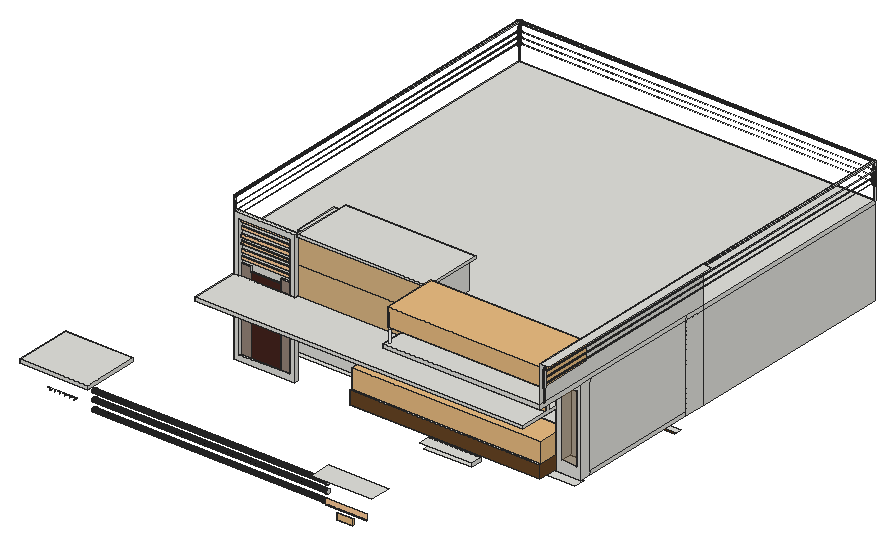
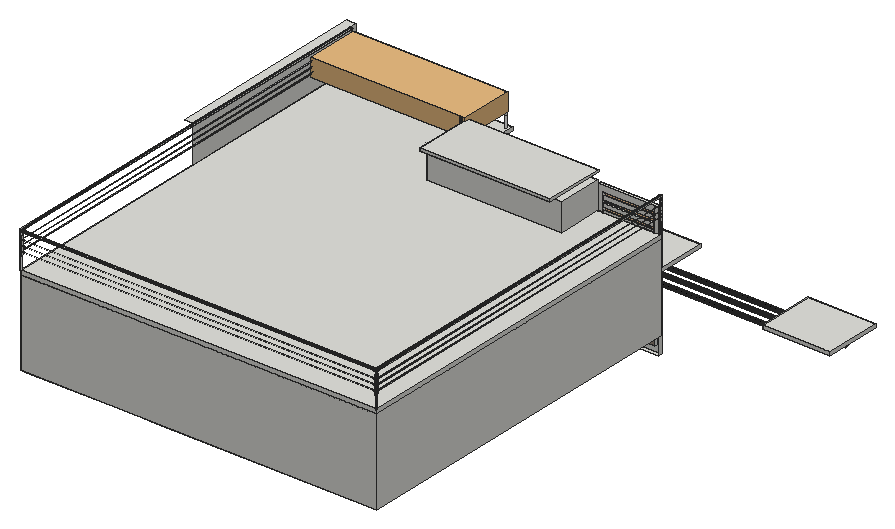
# SketchUp Ruby script. Lengths in millimetres.
U = 1.mm
M = Sketchup.active_model
def pt(a) = Geom::Point3d.new(a.map { |v| v * U })
def face(e, loops, mat)
  f = e.add_face(loops[0].map { |a| pt(a) })
  loops[1..].each { |l| e.add_face(l.map { |a| pt(a) }).erase! }
  f.material = f.back_material = mat if mat
  f
end
# faces: each face lists its corners as indices into pts; further lists are holes
def faces(e, pts, list, mat = nil) = list.each { |f| face(e, (f[0].is_a?(Array) ? f : [f]).map { |l| l.map { |i| pts[i] } }, mat) }
# xy, xz, yz: faces in a plane at the given z, y or x. An outline is a flat list of corners, or four numbers for a rectangle; further outlines are holes
def ring(l) = l.size == 4 ? [[l[0], l[1]], [l[2], l[1]], [l[2], l[3]], [l[0], l[3]]] : l.each_slice(2).to_a
def flat(e, list, mat, &to3) = list.each { |f| face(e, (f[0].is_a?(Array) ? f : [f]).map { |l| ring(l).map { |u, v| to3.(u, v) } }, mat) }
def xy(e, z, list, mat = nil) = flat(e, list, mat) { |x, y| [x, y, z] }
def xz(e, y, list, mat = nil) = flat(e, list, mat) { |x, z| [x, y, z] }
def yz(e, x, list, mat = nil) = flat(e, list, mat) { |y, z| [x, y, z] }
def lines(e, pts, list) = list.each { |a, b| e.add_line(pt(pts[a]), pt(pts[b])) }
# prism: a flat outline (further loops are holes) pulled along v
def prism(e, loops, v, mat = nil)
  f = face(e, loops, mat); d = Geom::Vector3d.new(v.map { |x| x * U })
  f.pushpull(f.normal.samedirection?(d) ? d.length : -d.length)
end
def box(e, o, s, mat = nil) = prism(e, [[o, [o[0] + s[0], o[1], o[2]], [o[0] + s[0], o[1] + s[1], o[2]], [o[0], o[1] + s[1], o[2]]]], [0, 0, s[2]], mat)
def at(x, y, z, deg = 0) = Geom::Transformation.translation(pt([x, y, z])) * Geom::Transformation.rotation(ORIGIN, Z_AXIS, deg.degrees)
def axes(o, x, y, z) = Geom::Transformation.new([*x, 0, *y, 0, *z, 0, *pt(o).to_a, 1])
def part(name) = M.definitions.add(name)
# library, detail: a bought-in or finely detailed component or shape, given as its bounding box
def library(name, o, s) = part(name).tap { |d| box(d.entities, o, s) }
def detail(e, o, s) = box(e.add_group.entities, o, s)
def put(e, d, t, mat = nil) = e.add_instance(d, t).tap { |i| i.material = mat if mat }
def group(e, t, mat = nil) = e.add_group.tap { |g| g.transformation = t; g.material = mat if mat }.entities
root = M.entities
M.materials.add("[Carpet Berber Multi]").color = [151, 134, 122]
M.materials.add("[Color B08]").color = [102, 25, 0]
M.materials.add("[Color C02]").color = [255, 204, 153]
M.materials.add("[Color C04]").color = [255, 153, 50]
M.materials.add("[Color C08]").color = [102, 51, 0]
M.materials.add("[Color M09]").color = [0, 0, 0]
M.materials.add("[Translucent Glass Blue]").color = [100, 149, 237]
M.materials["[Translucent Glass Blue]"].alpha = 0.5
M.materials.add("[Translucent Glass Gray]").color = [128, 100, 65]
M.materials["[Translucent Glass Gray]"].alpha = 0.5
M.materials.add("[Wallpaper Stripe]").color = [70, 36, 30]
M.materials.add("[Wallpaper Stripe]1").color = [222, 185, 133]
M.materials.add("[Wood Veneer 01]").color = [104, 70, 37]
M.materials.add("white").color = [255, 255, 255]
c1 = library("104",[25.7,0,0],[638.7,244.6,25.4])
c2 = library("Group\#3",[0,0,0],[7711.1,1233,787])
c3 = library("jali",[1080.3,825,0],[50,600,2550])
c4 = part("Ploe\#1")
box(c4.entities,[74615.6,-1815.5,7016.8],[50.1,12,1447.8],"white")
box(c4.entities,[74608.7,-1803.5,7559.7],[64,12,723.9])
box(c4.entities,[74608.6,-1827.5,7559.7],[64,12,723.9])
c5 = part("Group10\#1")
put(c5.entities,c4,at(0,0,0))
put(c5.entities,c4,at(149287.3,13184.4,0,-180))
c6 = part("Ploe")
prism(c6.entities,[[[68450.6,318.1,7016.8],[68500.5,315.7,7016.8],[68500,303.7,7016.8],[68450,306.1,7016.8]]],[0,0,1295.4],"white")
prism(c6.entities,[[[68443,306.4,7502.5],[68507,303.4,7502.5],[68506.4,291.4,7502.5],[68442.4,294.5,7502.5]]],[0,0,647.7])
prism(c6.entities,[[[68507.5,315.3,7502.5],[68443.6,318.4,7502.5],[68444.2,330.4,7502.5],[68508.1,327.3,7502.5]]],[0,0,647.7])
c7 = part("Group3\#1")
put(c7.entities,c6,at(0,0,0))
put(c7.entities,c6,at(21358.4,-51621,0,46.381))
put(c7.entities,c6,at(78256.3,-70215.3,0,92.762))
c8 = library("Group\#1",[0,0,0],[6327.3,2197.8,730.1])
c9 = part("Ploe\#2")
box(c9.entities,[74615.6,14974.9,7016.8],[12.1,50,1447.8],"white")
box(c9.entities,[74603.6,14967.9,7559.7],[12.1,64,723.9])
box(c9.entities,[74627.6,14967.9,7559.7],[12.1,64.1,723.9])
c10 = part("Group14\#1")
put(c10.entities,c9,at(0,0,0))
put(c10.entities,c9,at(134790.3,29993.9,0,-180))
c11 = part("Ploe\#3")
box(c11.entities,[60137.6,15012.9,7016.8],[50,12,1447.8],"white")
box(c11.entities,[60130.6,15000.9,7559.7],[64,12,723.9])
box(c11.entities,[60130.6,15024.9,7559.7],[64,12,723.9])
c12 = part("Group18\#1")
put(c12.entities,c11,at(0,0,0))
put(c12.entities,c11,at(120331.3,15534.9,0,-180))
xy(root,2146.4,[[6096.2,2705.1,7130.5,2730.5]])
xy(root,2222.2,[[6020.4,2705.1,7206.3,2730.5]])
xy(root,2265.6,[[17916.4,7006,19853.2,7467.9]])
xy(root,2395.6,[[19543.5,12344.7,21847.6,12573.3]])
xy(root,2420.1,[[17737,7006,19853.2,7467.9]])
xy(root,2527.5,[[22164,12344.7,23841.8,12522.5]],"[Color C08]")
xy(root,2590.3,[[9937.1,7320.3,12413.6,7467.9]])
xy(root,2627.4,[[22064.1,12344.7,23941.7,12573.3]])
xy(root,2802.3,[[10549.1,7393.3,11768.3,7467.9]])
xy(root,2830.6,[[10133,7320.3,12184.4,7320.3,12184.4,7393.3,11768.3,7393.3,11768.3,7467.9,10549.1,7467.9,10549.1,7393.3,10133,7393.3]])
xy(root,2994,[[5211.2,2308.2,5428.7,4629.3],[5428.7,2308.2,5561.2,2705.1],[5561.2,2308.2,5760.5,2705.1],[5760.5,2308.2,7761.5,2705.1],[7761.5,2308.2,7964.7,4629.3],
  [5428.7,4232.4,5779.6,4629.3],[5779.6,4232.4,7761.5,4629.3]])
xy(root,3053.2,[[16385.5,7006,24068.1,7467.9]])
xy(root,3141.7,[[17189.8,2189.2,19635.7,3052.8],[5211.2,2308.2,7964.7,4629.3]])
xy(root,3352.8,[[15925.7,7006,23273.7,7467.9],[23273.7,7006,24127.4,7467.9],[24127.4,7006,24317.2,7467.9],[19440.4,7467.9,24317.2,12344.7],[10067.8,7696.5,19211.8,12573.3],
  [19440.4,12344.7,19440.4,12573.3,24088.6,12573.3,24088.6,21945.9,24317.2,21945.9,24317.2,12344.7],[9839.2,12573.3,10067.8,16840.5],[10067.8,12573.3,10067.8,16840.5,19211.8,16840.5,19211.8,21717.3,19440.4,21717.3,19440.4,12573.3],[19440.4,12573.3,24088.6,21717.3],[9839.2,16840.5,19211.8,16840.5,19211.8,21717.3,18983.2,21717.3,18983.2,17069.1,9839.2,17069.1],
  [9839.2,17069.1,18983.2,21717.3],[9839.2,21717.3,18983.2,21945.9],[18983.2,21717.3,19440.4,21945.9],[19440.4,21717.3,24088.6,21945.9]])
xy(root,3388.1,[[15532.7,6218.6,23273.7,7467.9]])
xy(root,3497.3,[[15634.5,6372.7,23172,7467.9],[19430.1,7467.9,24317.2,7467.9,24317.2,12355.9,21589.7,12355.9,21589.7,12457.5,20354,12457.5,20354,12355.9,19430.1,12355.9],[10067.8,7696.5,19201.5,7696.5,19201.5,12584.5,24088.6,12584.5,24088.6,21717.3,10067.8,21717.3],[20267,12355.9,20354,12355.9,20354,12457.5,21589.7,12457.5,21589.7,12355.9,21676.7,12355.9,21676.7,12584.5,20267,12584.5]])
xy(root,3807.3,[[23509.7,7006,24144.7,14041.8]])
xy(root,3920.5,[[15532.7,6218.6,23273.7,6218.6,23273.7,7467.9,23172,7467.9,23172,6372.7,15634.5,6372.7,15634.5,7467.9,15532.7,7467.9]])
xy(root,3962.4,[[16385.5,7404.4,17916.4,7467.9]])
xy(root,3995.4,[[16418.5,7404.4,16866.2,7467.9],[16893.9,7404.4,17443.7,7467.9],[17471.8,7404.4,17883.4,7467.9]],"[Color M09]")
xy(root,4317.4,[[16418.5,7404.4,16866.2,7467.9],[16893.9,7404.4,17443.7,7467.9],[17471.8,7404.4,17883.4,7467.9]])
xy(root,4343.1,[[16418.5,7404.4,16866.2,7467.9],[16893.9,7404.4,17443.7,7467.9],[17471.8,7404.4,17883.4,7467.9]],"[Color M09]")
xy(root,4491.4,[[22151.9,12355.9,23918.8,12584.5]])
xy(root,4663.1,[[21219.3,12355.9,21498.7,12457.5]],"[Color M09]")
xy(root,4739.3,[[21219.3,12355.9,21498.7,12457.5]],"[Color M09]")
xy(root,5021.4,[[16418.5,7404.4,16866.2,7467.9],[16893.9,7404.4,17443.7,7467.9],[17471.8,7404.4,17883.4,7467.9]])
xy(root,5045.6,[[16418.5,7404.4,16866.2,7467.9],[16893.9,7404.4,17443.7,7467.9],[17471.8,7404.4,17883.4,7467.9]])
xy(root,5453.4,[[16418.5,7404.4,16866.2,7467.9],[16893.9,7404.4,17443.7,7467.9],[17471.8,7404.4,17883.4,7467.9]])
xy(root,5486.4,[[16385.5,7404.4,17916.4,7467.9]])
xy(root,5591.3,[[9914.3,5335.9,9914.3,7320.3,12413.6,7320.3,12413.6,7467.9,23273.7,7467.9,23273.7,5335.9]])
xy(root,5602.6,[[22151.9,12355.9,23918.8,12584.5]])
xy(root,5691.2,[[20354,12355.9,21589.7,12457.5]],"[Color C08]")
xy(root,5716.7,[[9914.3,5335.9,23273.7,5335.9,23273.7,6566.4,17916.4,6566.4,17916.4,6682.1,23273.7,6682.1,23273.7,7467.9,12413.6,7467.9,12413.6,7320.3,9914.3,7320.3],[19430.1,7467.9,23273.7,7527.9]])
xy(root,5778.2,[[20267,12355.9,21676.7,12584.5]])
xy(root,5962.4,[[10549.1,7393.3,11768.3,7467.9]])
xy(root,6145.2,[[10133,7393.3,10549.1,7467.9],[11768.3,7393.3,12184.4,7467.9]])
xy(root,6273.4,[[10133,7396.5,12184.4,7467.9]])
xy(root,6392.5,[[10133,7396.5,12184.4,7467.9]])
xy(root,6548.2,[[10133,7396.5,12184.4,7467.9]])
xy(root,6568,[[23509.7,7006,24144.7,14041.8]])
xy(root,6667.3,[[10133,7396.5,12184.4,7467.9]])
xy(root,6823,[[10133,7396.5,12184.4,7467.9]])
xy(root,6850.1,[[17916.4,6566.4,23273.7,6682.1],[23273.7,7006,24127.4,7467.9],[24127.4,7006,24317.2,7467.9],[10133,7396.5,10133,7467.9,10067.8,7467.9,10067.8,7696.5,19201.5,7696.5,19201.5,7467.9,12184.4,7467.9,12184.4,7396.5],[19201.5,7467.9,23273.7,7467.9,23273.7,7527.9,19430.1,7527.9,19430.1,12355.9,24317.2,12355.9,24317.2,12584.5,19201.5,12584.5],
  [23273.7,7467.9,23273.7,7527.9,19430.1,7527.9,19430.1,12355.9,24317.2,12355.9,24317.2,7467.9],[10067.8,7696.5,19201.5,21717.3],[19201.5,12584.5,24088.6,21717.3],[24088.6,12584.5,24317.2,21717.3],[10067.8,21717.3,19201.5,21945.9],
  [19201.5,21717.3,24317.2,21945.9]])
xy(root,6850.1,[[17916.4,4921.6,17916.4,6566.4,23273.7,6566.4,23273.7,6682.1,17916.4,6682.1,17916.4,7467.9,23273.7,7467.9,23273.7,7006,24317.2,7006,24317.2,4921.6]],"[Color B08]")
xy(root,6942.1,[[10133,7396.5,12184.4,7467.9]])
xy(root,7097.8,[[10133,7396.5,12184.4,7467.9]])
xy(root,7216.9,[[10133,7396.5,12184.4,7467.9]])
xy(root,7372.6,[[10133,7391.7,12184.4,7467.9]])
xy(root,7491.7,[[10133,7391.7,12184.4,7467.9]])
xy(root,7647.4,[[10133,7407.6,12184.4,7467.9]])
xy(root,7766.6,[[10133,7320.3,12184.4,7407.6],[10133,7407.6,12184.4,7467.9]])
xy(root,8001,[[9937.1,7320.3,12413.6,7467.9]])
xy(root,8129.6,[[12697.5,7072.7,17916.4,7467.9],[17916.4,7072.7,18021.2,9525.3],[12413.6,7467.9,12697.5,9311],[12697.5,9311,17916.4,9525.3]])
xy(root,8224.8,[[12697.5,7072.7,18021.2,9525.3]])
xy(root,8532.8,[[24317.2,4921.6,24679,13178.8]])
xz(root,2189.2,[[17767.7,2287.5,19436.2,2331.1],[17767.7,2331.1,19436.2,2536.5]],"[Color C02]")
xz(root,2308.2,[[5211.2,2994,7964.7,3141.7]])
xz(root,4629.3,[[5211.2,2994,7964.7,3141.7]])
xz(root,4921.6,[[17916.4,6850.1,24317.2,7016.8]])
xz(root,5335.9,[[9914.3,5591.3,23273.7,5716.7]])
xz(root,6218.6,[[15532.7,3388.1,23273.7,3920.5]],"[Wood Veneer 01]")
xz(root,6372.7,[[15634.5,3497.3,23172,3920.5]])
xz(root,6566.4,[[17916.4,5716.7,23273.7,6850.1]])
xz(root,6682.1,[[17916.4,5716.7,23273.7,6850.1]])
xz(root,7006,[[[23273.7,3352.8,24317.2,6850.1],[23509.7,3807.3,24144.7,6568]]])
xz(root,7006,[[23509.7,3807.3,24144.7,6568]],"[Translucent Glass Gray]")
xz(root,7072.7,[[12697.5,8129.6,18021.2,8224.8]])
xz(root,7320.3,[[9937.1,2590.3,12413.6,2590.3,12413.6,5591.3,12184.4,5591.3,12184.4,2830.6,10133,2830.6,10133,5591.3,9937.1,5591.3],[9914.3,5591.3,9937.1,5716.7],[9937.1,5591.3,10133,5716.7],[10133,5591.3,12184.4,5716.7],[12184.4,5591.3,12413.6,5716.7],
  [9937.1,5716.7,10133,5716.7,10133,7766.6,12184.4,7766.6,12184.4,5716.7,12413.6,5716.7,12413.6,8001,9937.1,8001]])
xz(root,7391.7,[[10133,7372.6,12184.4,7491.7]],"[Color C02]")
xz(root,7393.3,[[10133,2830.6,10549.1,6145.2],[11768.3,2830.6,12184.4,6145.2]],"[Carpet Berber Multi]")
xz(root,7393.3,[[10549.1,2802.3,11768.3,5962.4]],"[Wallpaper Stripe]")
xz(root,7396.5,[[10133,6273.4,12184.4,6392.5],[10133,6548.2,12184.4,6667.3],[10133,6823,12184.4,6850.1],[10133,6850.1,12184.4,6942.1],[10133,7097.8,12184.4,7216.9]],"[Color C02]")
xz(root,7404.4,[[[16385.5,3962.4,17916.4,5486.4],[16418.5,3995.4,17883.4,5453.4]],[[16866.2,3995.4,16893.9,3995.4,16893.9,4317.4,17443.7,4317.4,17443.7,3995.4,17471.8,3995.4,17471.8,4317.4,17883.4,4317.4,17883.4,4343.1,17471.8,4343.1,17471.8,5021.4,17883.4,5021.4,17883.4,5045.6,17471.8,5045.6,17471.8,5453.4,17443.7,5453.4,17443.7,5045.6,16893.9,5045.6,16893.9,5453.4,16866.2,5453.4,16866.2,5045.6,16418.5,5045.6,16418.5,5021.4,16866.2,5021.4,16866.2,4343.1,16418.5,4343.1,16418.5,4317.4,16866.2,4317.4],[16893.9,4343.1,17443.7,5021.4]]],"[Color M09]")
xz(root,7407.6,[[10133,7647.4,12184.4,7766.6]],"[Color C02]")
xz(root,7467.9,[[17916.4,2133.6,19440.4,2265.6],[17737,2265.6,17916.4,2420.1],[17916.4,2265.6,19440.4,2420.1],[19440.4,2265.6,19853.2,2420.1],[10549.1,2802.3,11768.3,2830.6],
  [11768.3,2830.6,12184.4,6145.2],[23273.7,3352.8,24127.4,3497.3],[24127.4,3352.8,24317.2,3497.3],[23172,3497.3,23273.7,3920.5],[23273.7,3497.3,24127.4,6850.1],
  [24127.4,3497.3,24317.2,6850.1],[19430.1,5591.3,23273.7,5716.7],[10549.1,5962.4,11768.3,5962.4,11768.3,6145.2,12184.4,6145.2,12184.4,6273.4,10133,6273.4,10133,6145.2,10549.1,6145.2],[10133,6392.5,12184.4,6548.2],[10133,6667.3,12184.4,6823],
  [9839.2,6850.1,9937.1,6850.1,9937.1,7016.7,9839.2,7016.8],[10067.8,6850.1,10133,7016.7],[12184.4,6850.1,12413.6,7016.7],[10133,6942.1,12184.4,7016.7],[9937.1,7016.7,10067.8,8001],
  [10067.8,7016.7,10067.8,8001,12413.6,8001,12413.6,7016.7,12184.4,7016.7,12184.4,7766.6,10133,7766.6,10133,7016.7],[10133,7016.7,12184.4,7097.8],[10133,7216.9,12184.4,7372.6],[10133,7491.7,12184.4,7647.4]])
xz(root,7467.9,[[16418.5,3995.4,16866.2,4317.4],[16893.9,3995.4,17443.7,4317.4],[17471.8,3995.4,17883.4,4317.4],[16418.5,4343.1,16866.2,5021.4],[16893.9,4343.1,17443.7,5021.4],
  [17471.8,4343.1,17883.4,5021.4],[16418.5,5045.6,16866.2,5453.4],[16893.9,5045.6,17443.7,5453.4],[17471.8,5045.6,17883.4,5453.4]],"[Translucent Glass Gray]")
xz(root,7467.9,[[12413.6,5716.7,23273.7,6850.1],[12413.6,6850.1,17916.4,8129.6]],"[Wallpaper Stripe]1")
xz(root,7527.9,[[19430.1,5716.7,23273.7,6850.1]])
xz(root,7696.5,[[10067.8,3497.3,19201.5,6850.1]])
xz(root,9311,[[12413.6,7016.7,12413.6,8129.6,17916.4,8129.6,17916.4,7016.8]])
xz(root,9525.3,[[12697.5,8129.6,18021.2,8224.8]])
xz(root,12355.9,[[[19430.1,3497.3,20267,3497.3,20267,5778.2,21676.7,5778.2,21676.7,3497.3,24317.2,3497.3,24317.2,6850.1,19430.1,6850.1],[22151.9,4491.4,23918.8,5602.6]]])
xz(root,12355.9,[[20267,3497.3,20354,3497.3,20354,5691.2,21589.7,5691.2,21589.7,3497.3,21676.7,3497.3,21676.7,5778.2,20267,5778.2],[21219.3,4663.1,21498.7,4739.3]],"[Color M09]")
xz(root,12457.5,[[20399.6,3497.3,20528.6,5691.2],[20595.8,3497.3,20742.9,5691.2]],"[Color C04]")
xz(root,12457.5,[[20354,3497.3,20399.6,5691.2],[20528.6,3497.3,20595.8,5691.2],[[20742.9,3497.3,21589.7,5691.2],[21219.3,4663.1,21498.7,4739.3]]],"[Color C08]")
xz(root,12584.5,[[[19201.5,3497.3,19201.5,6850.1,24088.6,6850.1,24088.6,3497.3,21676.7,3497.3,21676.7,5778.2,20267,5778.2,20267,3497.3],[22151.9,4491.4,23918.8,5602.6]]])
xz(root,14041.8,[[23509.7,3807.3,24144.7,6568]])
xz(root,21717.3,[[10067.8,3497.3,24088.6,6850.1]])
xz(root,21945.9,[[9839.2,3352.8,24317.2,6850.1],[9839.2,6850.1,24317.2,7016.8]])
yz(root,5211.2,[[2308.2,2994,4629.3,3141.7]])
yz(root,7964.7,[[2308.2,2994,4629.3,3141.7]])
yz(root,9839.2,[[7467.9,3352.8,21945.9,6850.1],[7467.9,6850.1,21945.9,7016.8]])
yz(root,9914.3,[[5335.9,5591.3,7320.3,5716.7]])
yz(root,9937.1,[[7320.3,2590.3,7467.9,8001]])
yz(root,10067.8,[[7696.5,3497.3,21717.3,6850.1]])
yz(root,10133,[[7320.3,2830.6,7393.3,2830.6,7393.3,6145.2,7467.9,6145.2,7467.9,6273.4,7396.5,6273.4,7396.5,6392.5,7467.9,6392.5,7467.9,6548.2,7396.5,6548.2,7396.5,6667.3,7467.9,6667.3,7467.9,6823,7396.5,6823,7396.5,6942.1,7467.9,6942.1,7467.9,7097.8,7396.5,7097.8,7396.5,7216.9,7467.9,7216.9,7467.9,7372.6,7391.7,7372.6,7391.7,7491.7,7467.9,7491.7,7467.9,7647.4,7407.6,7647.4,7407.6,7766.6,7320.3,7766.6],[7396.5,6850.1,7467.9,6942.1],[7396.5,7097.8,7467.9,7216.9],[7391.7,7372.6,7467.9,7491.7],[7407.6,7647.4,7467.9,7766.6]])
yz(root,10549.1,[[7393.3,2802.3,7467.9,2830.6],[7393.3,5962.4,7467.9,6145.2]])
yz(root,11768.3,[[7393.3,2802.3,7467.9,2830.6],[7393.3,2830.6,7467.9,5962.4],[7393.3,5962.4,7467.9,6145.2]])
yz(root,12184.4,[[7320.3,2830.6,7320.3,7766.6,7407.6,7766.6,7407.6,7647.4,7467.9,7647.4,7467.9,7491.7,7391.7,7491.7,7391.7,7372.6,7467.9,7372.6,7467.9,7216.9,7396.5,7216.9,7396.5,7097.8,7467.9,7097.8,7467.9,6942.1,7396.5,6942.1,7396.5,6823,7467.9,6823,7467.9,6667.3,7396.5,6667.3,7396.5,6548.2,7467.9,6548.2,7467.9,6392.5,7396.5,6392.5,7396.5,6273.4,7467.9,6273.4,7467.9,6145.2,7393.3,6145.2,7393.3,2830.6],[7393.3,2830.6,7467.9,6145.2],[7396.5,6850.1,7467.9,6942.1],[7396.5,7097.8,7467.9,7216.9],[7391.7,7372.6,7467.9,7491.7],
  [7407.6,7647.4,7467.9,7766.6]])
yz(root,12413.6,[[7320.3,2590.3,7467.9,5591.3],[7320.3,5591.3,7467.9,5716.7],[7320.3,5716.7,7467.9,8001],[7467.9,7016.7,9311,8129.6]])
yz(root,12697.5,[[7072.7,8129.6,9525.3,8224.8]])
yz(root,15532.7,[[6218.6,3388.1,7467.9,3920.5]],"[Wood Veneer 01]")
yz(root,15634.5,[[6372.7,3497.3,7366.2,3920.5],[7366.2,3497.3,7467.9,3920.5]])
yz(root,16385.5,[[7404.4,3962.4,7467.9,5486.4]],"[Color M09]")
yz(root,16418.5,[[7404.4,3995.4,7467.9,4317.4],[7404.4,4343.1,7467.9,5021.4],[7404.4,5045.6,7467.9,5453.4]])
yz(root,16866.2,[[7404.4,3995.4,7467.9,4317.4],[7404.4,4343.1,7467.9,5021.4],[7404.4,5045.6,7467.9,5453.4]],"[Color M09]")
yz(root,16893.9,[[7404.4,3995.4,7467.9,4317.4],[7404.4,5045.6,7467.9,5453.4]])
yz(root,16893.9,[[7404.4,4343.1,7467.9,5021.4]],"[Color M09]")
yz(root,17334.1,[[2877.4,2234.1,2897.1,2236.7,2915.5,2244.3,2931.2,2256.5,2943.3,2272.2,2951,2290.6,2953.6,2310.3,2951,2330.1,2943.3,2348.4,2931.2,2364.2,2915.5,2376.3,2897.1,2383.9,2877.4,2386.5,2857.6,2383.9,2839.3,2376.3,2823.5,2364.2,2811.4,2348.4,2803.7,2330.1,2801.2,2310.3,2803.7,2290.6,2811.4,2272.2,2823.5,2256.5,2839.3,2244.3,2857.6,2236.7],[2877.4,2559.6,2897.1,2562.2,2915.5,2569.8,2931.2,2581.9,2943.3,2597.7,2951,2616.1,2953.6,2635.8,2951,2655.5,2943.3,2673.9,2931.2,2689.7,2915.5,2701.8,2897.1,2709.4,2877.4,2712,2857.6,2709.4,2839.3,2701.8,2823.5,2689.7,2811.4,2673.9,2803.7,2655.5,2801.2,2635.8,2803.7,2616.1,2811.4,2597.7,2823.5,2581.9,2839.3,2569.8,2857.6,2562.2]])
yz(root,17443.7,[[7404.4,3995.4,7467.9,4317.4],[7404.4,4343.1,7467.9,5021.4],[7404.4,5045.6,7467.9,5453.4]],"[Color M09]")
yz(root,17471.8,[[7404.4,3995.4,7467.9,4317.4],[7404.4,5045.6,7467.9,5453.4]])
yz(root,17471.8,[[7404.4,4343.1,7467.9,5021.4]],"[Color M09]")
yz(root,17883.4,[[7404.4,3995.4,7467.9,4317.4],[7404.4,4343.1,7467.9,5021.4],[7404.4,5045.6,7467.9,5453.4]],"[Color M09]")
yz(root,17916.4,[[7404.4,3962.4,7467.9,5486.4],[6566.4,5716.7,6682.1,6850.1],[4921.6,6850.1,7467.9,7016.8],[7467.9,7016.8,9311,8129.6]])
yz(root,18021.2,[[7072.7,8129.6,9525.3,8224.8]])
yz(root,19201.5,[[7696.5,3497.3,12584.5,6850.1]])
yz(root,19430.1,[[7467.9,3497.3,7527.9,5716.7],[7527.9,3497.3,12355.9,6850.1]])
yz(root,19853.2,[[7006,2265.6,7467.9,2420.1]])
yz(root,20267,[[12355.9,3497.3,12584.5,5778.2]])
yz(root,20354,[[12355.9,3497.3,12457.5,5691.2]],"[Color C08]")
yz(root,21219.3,[[12355.9,4663.1,12457.5,4739.3]],"[Color M09]")
yz(root,21498.7,[[12355.9,4663.1,12457.5,4739.3]],"[Color M09]")
yz(root,21589.7,[[12355.9,3497.3,12457.5,5691.2]],"[Color C08]")
yz(root,21676.7,[[12355.9,3497.3,12584.5,5778.2]])
yz(root,22151.9,[[12355.9,4491.4,12584.5,5602.6]])
yz(root,23172,[[6372.7,3497.3,7467.9,3920.5]])
yz(root,23273.7,[[7006,3352.8,7467.9,3388.1],[7006,3388.1,7467.9,3920.5],[7006,3920.5,7467.9,5591.3],[5335.9,5591.3,7006,5591.3,7006,5716.7,6682.1,5716.7,6682.1,6850.1,6566.4,6850.1,6566.4,5716.7,5335.9,5716.7],[7006,5591.3,7467.9,5716.7],
  [7006,5716.7,7467.9,6850.1],[7467.9,5716.7,7527.9,6850.1]])
yz(root,23273.7,[[6218.6,3388.1,7006,3920.5]],"[Wood Veneer 01]")
yz(root,23509.7,[[7006,3807.3,14041.8,6568]])
yz(root,23918.8,[[12355.9,4491.4,12584.5,5602.6]])
yz(root,24088.6,[[12584.5,3497.3,21717.3,6850.1]])
yz(root,24144.7,[[7006,3807.3,14041.8,6568]])
yz(root,24317.2,[[7006,3352.8,7467.9,6850.1],[7467.9,3352.8,12344.7,3497.3],[12344.7,3352.8,12344.7,3497.3,12355.9,3497.3,12355.9,6850.1,13178.8,6850.1,13178.8,3352.8],[13178.8,3352.8,21945.9,6850.1],[7467.9,3497.3,12344.7,6850.1],
  [12344.7,3497.3,12355.9,6850.1],[4921.6,6850.1,12344.7,7016.8],[12344.7,6850.1,13178.8,7016.8],[13178.8,6850.1,21945.9,7016.8],[4921.6,7016.8,13178.8,8532.8]])
p = [[7761.5,2857.6,1873.2],[7761.5,2877.4,1870.6],[17189.8,2877.4,1870.6],[17189.8,2857.6,1873.2],[7761.5,2897.1,1873.2],[17189.8,2897.1,1873.2],
  [7761.5,2839.3,1880.8],[17189.8,2839.3,1880.8],[7761.5,2915.5,1880.8],[17189.8,2915.5,1880.8],[7761.5,2823.5,1892.9],[17189.8,2823.5,1892.9],
  [7761.5,2931.2,1892.9],[17189.8,2931.2,1892.9],[7761.5,2811.4,1908.7],[17189.8,2811.4,1908.7],[7761.5,2943.3,1908.7],[17189.8,2943.3,1908.7],
  [7761.5,2803.7,1927.1],[17189.8,2803.7,1927.1],[7761.5,2951,1927.1],[17189.8,2951,1927.1],[7761.5,2801.2,1946.8],[17189.8,2801.2,1946.8],
  [7761.5,2953.6,1946.8],[17189.8,2953.6,1946.8],[7761.5,2803.7,1966.5],[17189.8,2803.7,1966.5],[7761.5,2951,1966.5],[17189.8,2951,1966.5],
  [7761.5,2811.4,1984.9],[17189.8,2811.4,1984.9],[7761.5,2943.3,1984.9],[17189.8,2943.3,1984.9],[7761.5,2823.5,2000.7],[17189.8,2823.5,2000.7],
  [7761.5,2931.2,2000.7],[17189.8,2931.2,2000.7],[7761.5,2839.3,2012.8],[17189.8,2839.3,2012.8],[7761.5,2915.5,2012.8],[17189.8,2915.5,2012.8],
  [7761.5,2857.6,2020.4],[17189.8,2857.6,2020.4],[7761.5,2897.1,2020.4],[17189.8,2897.1,2020.4],[7761.5,2877.4,2023],[17189.8,2877.4,2023],
  [7761.5,2857.6,2236.7],[7761.5,2877.4,2234.1],[17334.1,2877.4,2234.1],[17334.1,2857.6,2236.7],[7761.5,2897.1,2236.7],[17334.1,2897.1,2236.7],
  [7761.5,2839.3,2244.3],[17334.1,2839.3,2244.3],[7761.5,2915.5,2244.3],[17334.1,2915.5,2244.3],[7761.5,2823.5,2256.5],[17334.1,2823.5,2256.5],
  [7761.5,2931.2,2256.5],[17334.1,2931.2,2256.5],[7761.5,2811.4,2272.2],[17334.1,2811.4,2272.2],[7761.5,2943.3,2272.2],[17334.1,2943.3,2272.2],
  [7761.5,2803.7,2290.6],[17334.1,2803.7,2290.6],[7761.5,2951,2290.6],[17334.1,2951,2290.6],[7761.5,2801.2,2310.3],[17334.1,2801.2,2310.3],
  [7761.5,2953.6,2310.3],[17334.1,2953.6,2310.3],[7761.5,2803.7,2330.1],[17334.1,2803.7,2330.1],[7761.5,2951,2330.1],[17334.1,2951,2330.1],
  [7761.5,2811.4,2348.4],[17334.1,2811.4,2348.4],[7761.5,2943.3,2348.4],[17334.1,2943.3,2348.4],[7761.5,2823.5,2364.2],[17334.1,2823.5,2364.2],
  [7761.5,2931.2,2364.2],[17334.1,2931.2,2364.2],[7761.5,2839.3,2376.3],[17334.1,2839.3,2376.3],[7761.5,2915.5,2376.3],[17334.1,2915.5,2376.3],
  [7761.5,2857.6,2383.9],[17334.1,2857.6,2383.9],[7761.5,2897.1,2383.9],[17334.1,2897.1,2383.9],[7761.5,2877.4,2386.5],[17334.1,2877.4,2386.5],
  [7761.5,2857.6,2562.2],[7761.5,2877.4,2559.6],[17334.1,2877.4,2559.6],[17334.1,2857.6,2562.2],[7761.5,2897.1,2562.2],[17334.1,2897.1,2562.2],
  [7761.5,2839.3,2569.8],[17334.1,2839.3,2569.8],[7761.5,2915.5,2569.8],[17334.1,2915.5,2569.8],[7761.5,2823.5,2581.9],[17334.1,2823.5,2581.9],
  [7761.5,2931.2,2581.9],[17334.1,2931.2,2581.9],[7761.5,2811.4,2597.7],[17334.1,2811.4,2597.7],[7761.5,2943.3,2597.7],[17334.1,2943.3,2597.7],
  [7761.5,2803.7,2616.1],[17334.1,2803.7,2616.1],[7761.5,2951,2616.1],[17334.1,2951,2616.1],[7761.5,2801.2,2635.8],[17334.1,2801.2,2635.8],
  [7761.5,2953.6,2635.8],[17334.1,2953.6,2635.8],[7761.5,2803.7,2655.5],[17334.1,2803.7,2655.5],[7761.5,2951,2655.5],[17334.1,2951,2655.5],
  [7761.5,2811.4,2673.9],[17334.1,2811.4,2673.9],[7761.5,2943.3,2673.9],[17334.1,2943.3,2673.9],[7761.5,2823.5,2689.7],[17334.1,2823.5,2689.7],
  [7761.5,2931.2,2689.7],[17334.1,2931.2,2689.7],[7761.5,2839.3,2701.8],[17334.1,2839.3,2701.8],[7761.5,2915.5,2701.8],[17334.1,2915.5,2701.8],
  [7761.5,2857.6,2709.4],[17334.1,2857.6,2709.4],[7761.5,2897.1,2709.4],[17334.1,2897.1,2709.4],[7761.5,2877.4,2712],[17334.1,2877.4,2712],
  [23509.7,12337.6,5602.6],[22151.9,12355.9,5602.6],[22151.9,12355.9,4498.3],[23509.7,12337.6,4498.3],[22830.8,12346.8,4554.1],[22207.7,12355.2,4554.1],
  [22207.7,12355.2,5546.8],[22830.8,12346.8,5546.8],[23454,12338.4,5546.8],[23454,12338.4,4554.1],[10067.8,7467.9,7016.7],[10133,7467.9,7016.7],
  [12184.4,7467.9,7016.7],[12413.6,7467.9,7016.7],[12413.6,9311,7016.7],[17916.4,9311,7016.8],[17916.4,7467.9,7016.8],[17916.4,4921.6,7016.8],
  [24317.2,4921.6,7016.8],[24317.2,12344.7,7016.8],[24317.2,13178.8,7016.8],[24317.2,21945.9,7016.8],[9839.2,21945.9,7016.8],[9839.2,7467.9,7016.8],
  [9937.1,7467.9,7016.7],[19211.8,7696.5,3352.8],[19211.8,7467.9,3352.8],[10067.8,7467.9,3352.8],[10067.8,7696.5,3352.8],[19430.1,7527.9,6850.1],
  [19430.1,7467.9,7016.8]]
faces(root,p,[[0,1,2,3],[1,4,5,2],[6,0,3,7],[4,8,9,5],[10,6,7,11],[8,12,13,9],[14,10,11,15],[12,16,17,13],
  [18,14,15,19],[16,20,21,17],[22,18,19,23],[20,24,25,21],[26,22,23,27],[24,28,29,25],[30,26,27,31],[28,32,33,29],
  [34,30,31,35],[32,36,37,33],[38,34,35,39],[36,40,41,37],[42,38,39,43],[40,44,45,41],[46,42,43,47],[44,46,47,45],
  [48,49,50,51],[49,52,53,50],[54,48,51,55],[52,56,57,53],[58,54,55,59],[56,60,61,57],[62,58,59,63],[60,64,65,61],
  [66,62,63,67],[64,68,69,65],[70,66,67,71],[68,72,73,69],[74,70,71,75],[72,76,77,73],[78,74,75,79],[76,80,81,77],
  [82,78,79,83],[80,84,85,81],[86,82,83,87],[84,88,89,85],[90,86,87,91],[88,92,93,89],[94,90,91,95],[92,94,95,93],
  [96,97,98,99],[97,100,101,98],[102,96,99,103],[100,104,105,101],[106,102,103,107],[104,108,109,105],[110,106,107,111],[108,112,113,109],
  [114,110,111,115],[112,116,117,113],[118,114,115,119],[116,120,121,117],[122,118,119,123],[120,124,125,121],[126,122,123,127],[124,128,129,125],
  [130,126,127,131],[128,132,133,129],[134,130,131,135],[132,136,137,133],[138,134,135,139],[136,140,141,137],[142,138,139,143],[140,142,143,141],
  [[144,145,146,147],[148,149,150,151,152,153]]],"[Color M09]")
faces(root,p,[[152,151,148,153],[149,148,151,150]],"[Translucent Glass Gray]")
faces(root,p,[[154,155,156,157,158,159,160,161,162,163,164,165,166,167,168]])
lines(root,p,[[169,170],[171,172],[173,174]])
put(root,c1,axes([18230.7,2189.2,1926.7],[1,0,0],[0,0,1],[0,-1,0]))
put(root,c2,at(15543.6,6284.9,3920.5),"[Translucent Glass Blue]")
put(root,c3,axes([17916.4,5435.1,4158.3],[0,1,0],[0,0,1.88896],[2.1,0,0]))
g1 = group(root,at(24261.2,5124.5,7016.8))
put(g1,c5,at(-74590.7,1827.5,-7016.8))
g2 = group(g1,at(0,18,657.7))
prism(g2,[[[46.3,16803.5,7.4],[46,16803.5,10],[46.3,16803.5,12.6],[47.3,16803.5,15],[48.9,16803.5,17.1],[51,16803.5,18.7],[53.4,16803.5,19.7],[56,16803.5,20],[58.6,16803.5,19.7],[61,16803.5,18.7],[63.1,16803.4,17.1],[64.7,16803.4,15],[65.7,16803.4,12.6],[66,16803.4,10],[65.7,16803.4,7.4],[64.7,16803.4,5],[63.1,16803.4,2.9],[61,16803.5,1.3],[58.6,16803.5,0.3],[56,16803.5,0],[53.4,16803.5,0.3],[51,16803.5,1.3],[48.9,16803.5,2.9],[47.3,16803.5,5]]],[-6,-16803.4,0],"white")
prism(g2,[[[46.3,16803.5,224.6],[46,16803.5,227.2],[46.3,16803.5,229.8],[47.3,16803.5,232.2],[48.9,16803.5,234.2],[51,16803.5,235.8],[53.4,16803.5,236.8],[56,16803.5,237.2],[58.6,16803.5,236.8],[61,16803.5,235.8],[63.1,16803.4,234.2],[64.7,16803.4,232.2],[65.7,16803.4,229.8],[66,16803.4,227.2],[65.7,16803.4,224.6],[64.7,16803.4,222.2],[63.1,16803.4,220.1],[61,16803.5,218.5],[58.6,16803.5,217.5],[56,16803.5,217.2],[53.4,16803.5,217.5],[51,16803.5,218.5],[48.9,16803.5,220.1],[47.3,16803.5,222.2]]],[-6,-16803.4,0],"white")
prism(g2,[[[46.3,16803.5,441.8],[46,16803.5,444.3],[46.3,16803.5,446.9],[47.3,16803.5,449.3],[48.9,16803.5,451.4],[51,16803.5,453],[53.4,16803.5,454],[56,16803.5,454.3],[58.6,16803.5,454],[61,16803.5,453],[63.1,16803.4,451.4],[64.7,16803.4,449.3],[65.7,16803.4,446.9],[66,16803.4,444.3],[65.7,16803.4,441.8],[64.7,16803.4,439.3],[63.1,16803.4,437.3],[61,16803.5,435.7],[58.6,16803.5,434.7],[56,16803.5,434.3],[53.4,16803.5,434.7],[51,16803.5,435.7],[48.9,16803.5,437.3],[47.3,16803.5,439.3]]],[-6,-16803.4,0],"white")
xy(g2,770.1,[[0,0,100,0,6,16803.5],[100,0,106,16803.4,6,16803.5]])
xy(g2,810.1,[[15,0,21,16803.5,91,16803.4],[15,0,91,16803.4,85,0]])
xz(g2,0,[[0,770.1,0,795.1,15,810.1,85,810.1,100,795.1,100,770.1]])
p = [[0,0,795.1],[0,0,770.1],[6,16803.5,795.1],[6,16803.5,770.1],[100,0,770.1],[100,0,795.1],
  [106,16803.4,770.1],[106,16803.4,795.1],[91,16803.4,810.1],[21,16803.5,810.1],[15,0,810.1],[85,0,810.1]]
faces(g2,p,[[0,1,2],[2,1,3],[4,5,6],[6,5,7],[6,7,8,9,2,3],[10,0,9],[9,0,2],[5,11,7],
  [7,11,8]])
g3 = group(root,at(17989.9,5067.5,7016.8))
put(g3,c7,at(-68319.3,1884.5,-7016.8))
put(g3,c8,at(0,0,585.3))
g4 = group(root,at(9821.2,21895.9,7016.8))
put(g4,c10,at(-60150.6,-14943.9,-7016.8))
g5 = group(g4,at(18,0,657.7))
prism(g5,[[[14453,46,10],[14453,46.3,7.4],[14453,47.3,5],[14453,48.9,2.9],[14453,51,1.3],[14453,53.4,0.3],[14453,56,0],[14453,58.6,0.3],[14453,61,1.3],[14453,63.1,2.9],[14453,64.7,5],[14453,65.7,7.4],[14453,66,10],[14453,65.7,12.6],[14453,64.7,15],[14453,63.1,17.1],[14453,61,18.7],[14453,58.6,19.7],[14453,56,20],[14453,53.4,19.7],[14453,51,18.7],[14453,48.9,17.1],[14453,47.3,15],[14453,46.3,12.6]]],[-14453,-6,0],"white")
prism(g5,[[[14453,46,227.2],[14453,46.3,224.6],[14453,47.3,222.2],[14453,48.9,220.1],[14453,51,218.5],[14453,53.4,217.5],[14453,56,217.2],[14453,58.6,217.5],[14453,61,218.5],[14453,63.1,220.1],[14453,64.7,222.2],[14453,65.7,224.6],[14453,66,227.2],[14453,65.7,229.8],[14453,64.7,232.2],[14453,63.1,234.2],[14453,61,235.8],[14453,58.6,236.8],[14453,56,237.2],[14453,53.4,236.8],[14453,51,235.8],[14453,48.9,234.2],[14453,47.3,232.2],[14453,46.3,229.8]]],[-14453,-6,0],"white")
prism(g5,[[[14453,46,444.3],[14453,46.3,441.8],[14453,47.3,439.3],[14453,48.9,437.3],[14453,51,435.7],[14453,53.4,434.7],[14453,56,434.3],[14453,58.6,434.7],[14453,61,435.7],[14453,63.1,437.3],[14453,64.7,439.3],[14453,65.7,441.8],[14453,66,444.3],[14453,65.7,446.9],[14453,64.7,449.3],[14453,63.1,451.4],[14453,61,453],[14453,58.6,454],[14453,56,454.3],[14453,53.4,454],[14453,51,453],[14453,48.9,451.4],[14453,47.3,449.3],[14453,46.3,446.9]]],[-14453,-6,0],"white")
xy(g5,770.1,[[0,0,14453,106,0,100],[0,0,14453,6,14453,106]])
xy(g5,810.1,[[0,15,0,85,14453,21],[14453,21,0,85,14453,91]])
yz(g5,0,[[0,770.1,100,770.1,100,795.1,85,810.1,15,810.1,0,795.1]])
yz(g5,14453,[[6,770.1,6,795.1,21,810.1,91,810.1,106,795.1,106,770.1]])
p = [[14453,6,795.1],[14453,6,770.1],[0,0,795.1],[0,0,770.1],[14453,106,770.1],[14453,106,795.1],
  [0,100,770.1],[0,100,795.1],[0,15,810.1],[14453,21,810.1],[14453,91,810.1],[0,85,810.1]]
faces(g5,p,[[0,1,2],[2,1,3],[4,5,6],[6,5,7],[8,0,2],[9,0,8],[7,10,11],[5,10,7]])
g6 = group(root,at(9783.2,7449.9,7016.8))
put(g6,c12,at(-60112.6,-497.9,-7016.8))
g7 = group(g6,at(0,18,657.7))
prism(g7,[[[60,14503,10],[59.7,14503,7.4],[58.7,14503,5],[57.1,14503,2.9],[55,14503,1.3],[52.6,14503,0.3],[50,14503,0],[47.4,14503,0.3],[45,14503,1.3],[42.9,14503,2.9],[41.3,14503,5],[40.3,14503,7.4],[40,14503,10],[40.3,14503,12.6],[41.3,14503,15],[42.9,14503,17.1],[45,14503,18.7],[47.4,14503,19.7],[50,14503,20],[52.6,14503,19.7],[55,14503,18.7],[57.1,14503,17.1],[58.7,14503,15],[59.7,14503,12.6]]],[6,-14503,0],"white")
prism(g7,[[[60,14503,227.2],[59.7,14503,224.6],[58.7,14503,222.2],[57.1,14503,220.1],[55,14503,218.5],[52.6,14503,217.5],[50,14503,217.2],[47.4,14503,217.5],[45,14503,218.5],[42.9,14503,220.1],[41.3,14503,222.2],[40.3,14503,224.6],[40,14503,227.2],[40.3,14503,229.8],[41.3,14503,232.2],[42.9,14503,234.2],[45,14503,235.8],[47.4,14503,236.8],[50,14503,237.2],[52.6,14503,236.8],[55,14503,235.8],[57.1,14503,234.2],[58.7,14503,232.2],[59.7,14503,229.8]]],[6,-14503,0],"white")
prism(g7,[[[60,14503,444.3],[59.7,14503,441.8],[58.7,14503,439.3],[57.1,14503,437.3],[55,14503,435.7],[52.6,14503,434.7],[50,14503,434.3],[47.4,14503,434.7],[45,14503,435.7],[42.9,14503,437.3],[41.3,14503,439.3],[40.3,14503,441.8],[40,14503,444.3],[40.3,14503,446.9],[41.3,14503,449.3],[42.9,14503,451.4],[45,14503,453],[47.4,14503,454],[50,14503,454.3],[52.6,14503,454],[55,14503,453],[57.1,14503,451.4],[58.7,14503,449.3],[59.7,14503,446.9]]],[6,-14503,0],"white")
xy(g7,770.1,[[106,0,100,14503,0,14503],[6,0,106,0,0,14503]])
xy(g7,810.1,[[21,0,15,14503,85,14503],[21,0,85,14503,91,0]])
xz(g7,0,[[6,770.1,6,795.1,21,810.1,91,810.1,106,795.1,106,770.1]])
xz(g7,14503,[[0,770.1,100,770.1,100,795.1,85,810.1,15,810.1,0,795.1]])
p = [[0,14503,770.1],[0,14503,795.1],[6,0,770.1],[6,0,795.1],[100,14503,795.1],[100,14503,770.1],
  [106,0,795.1],[106,0,770.1],[15,14503,810.1],[21,0,810.1],[85,14503,810.1],[91,0,810.1]]
faces(g7,p,[[0,1,2],[2,1,3],[4,5,6],[6,5,7],[1,8,3],[3,8,9],[10,4,11],[11,4,6]])
